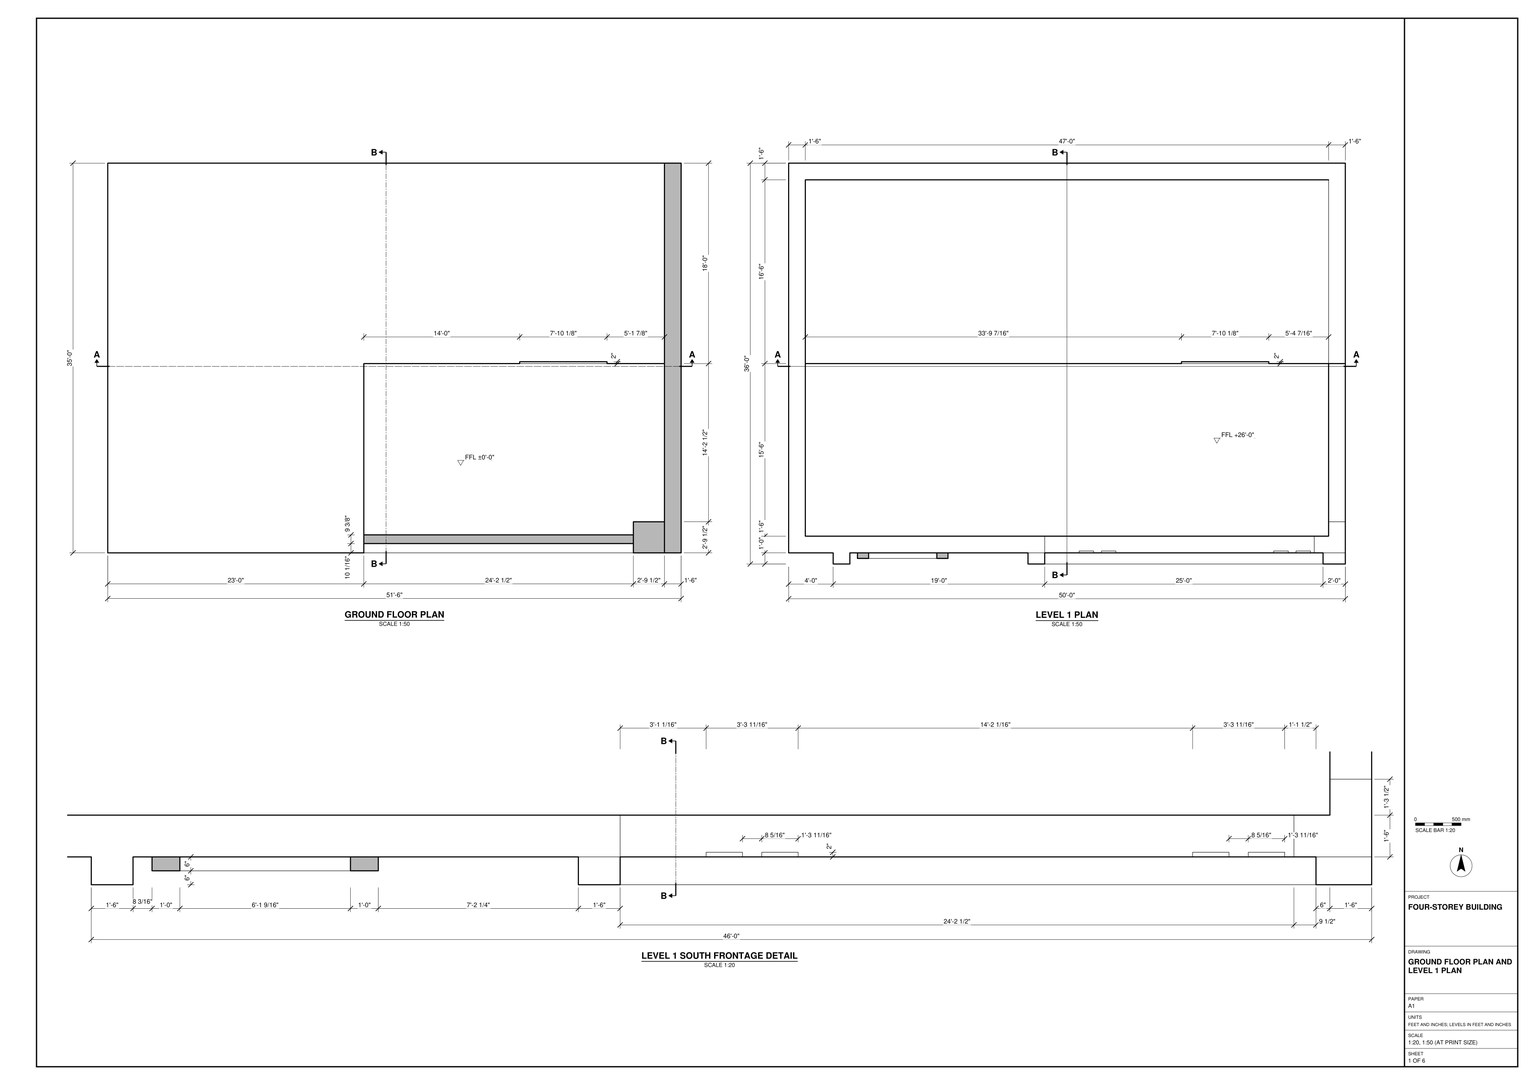
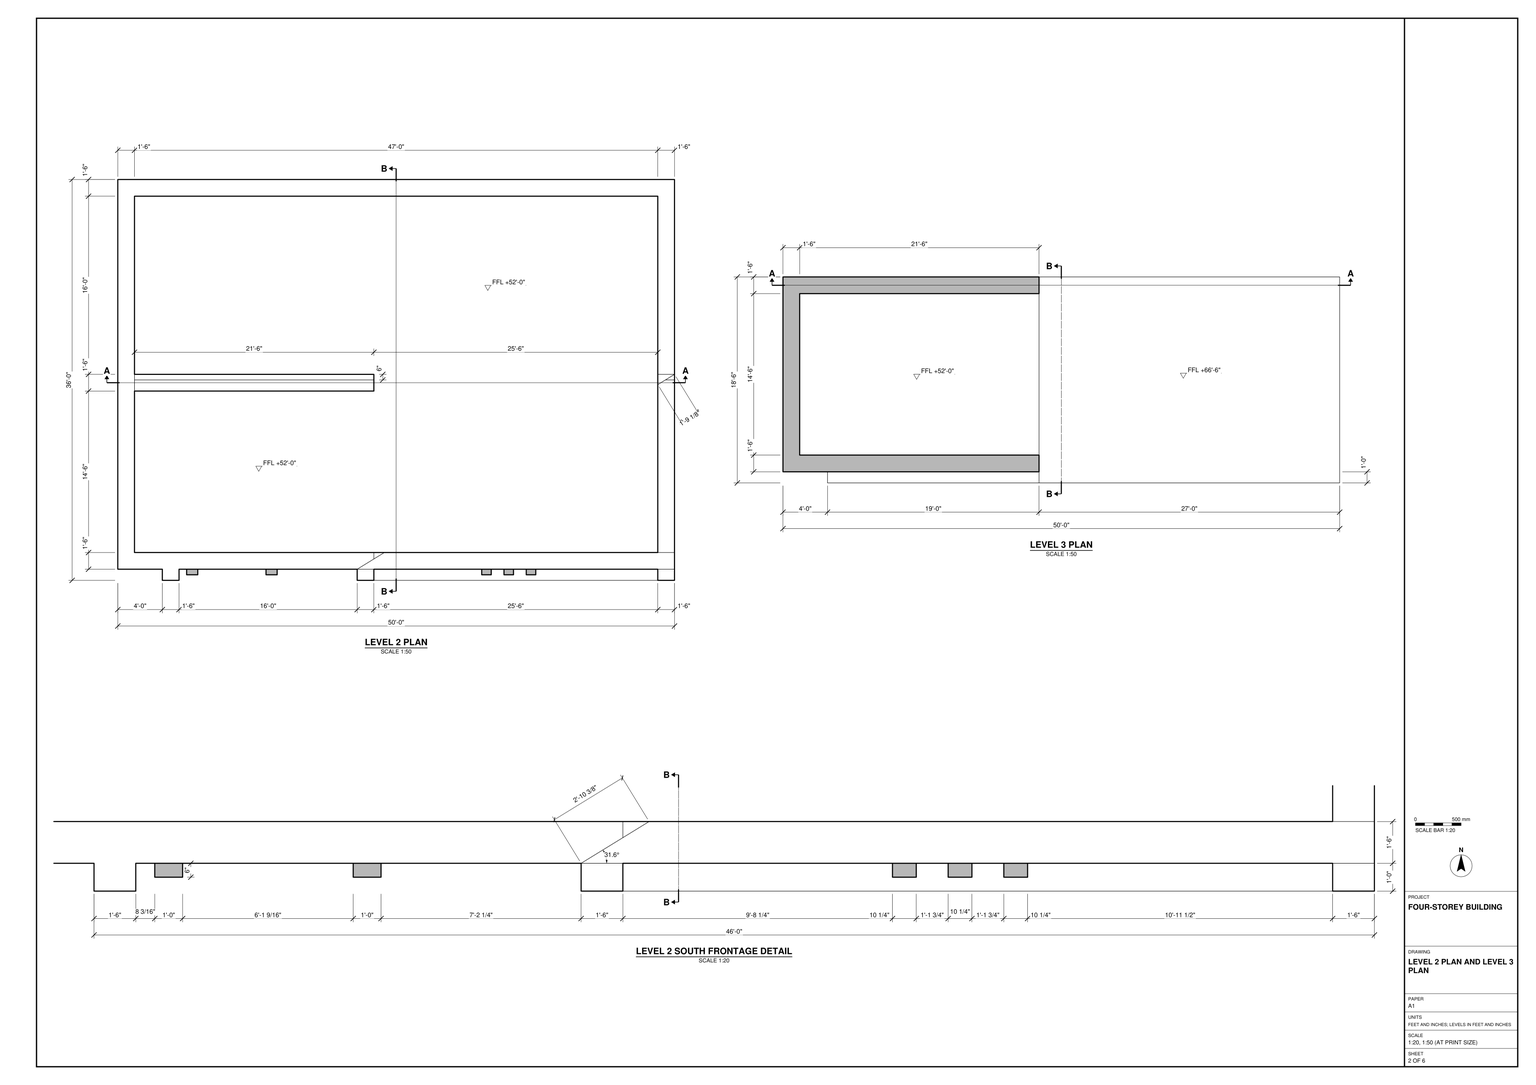
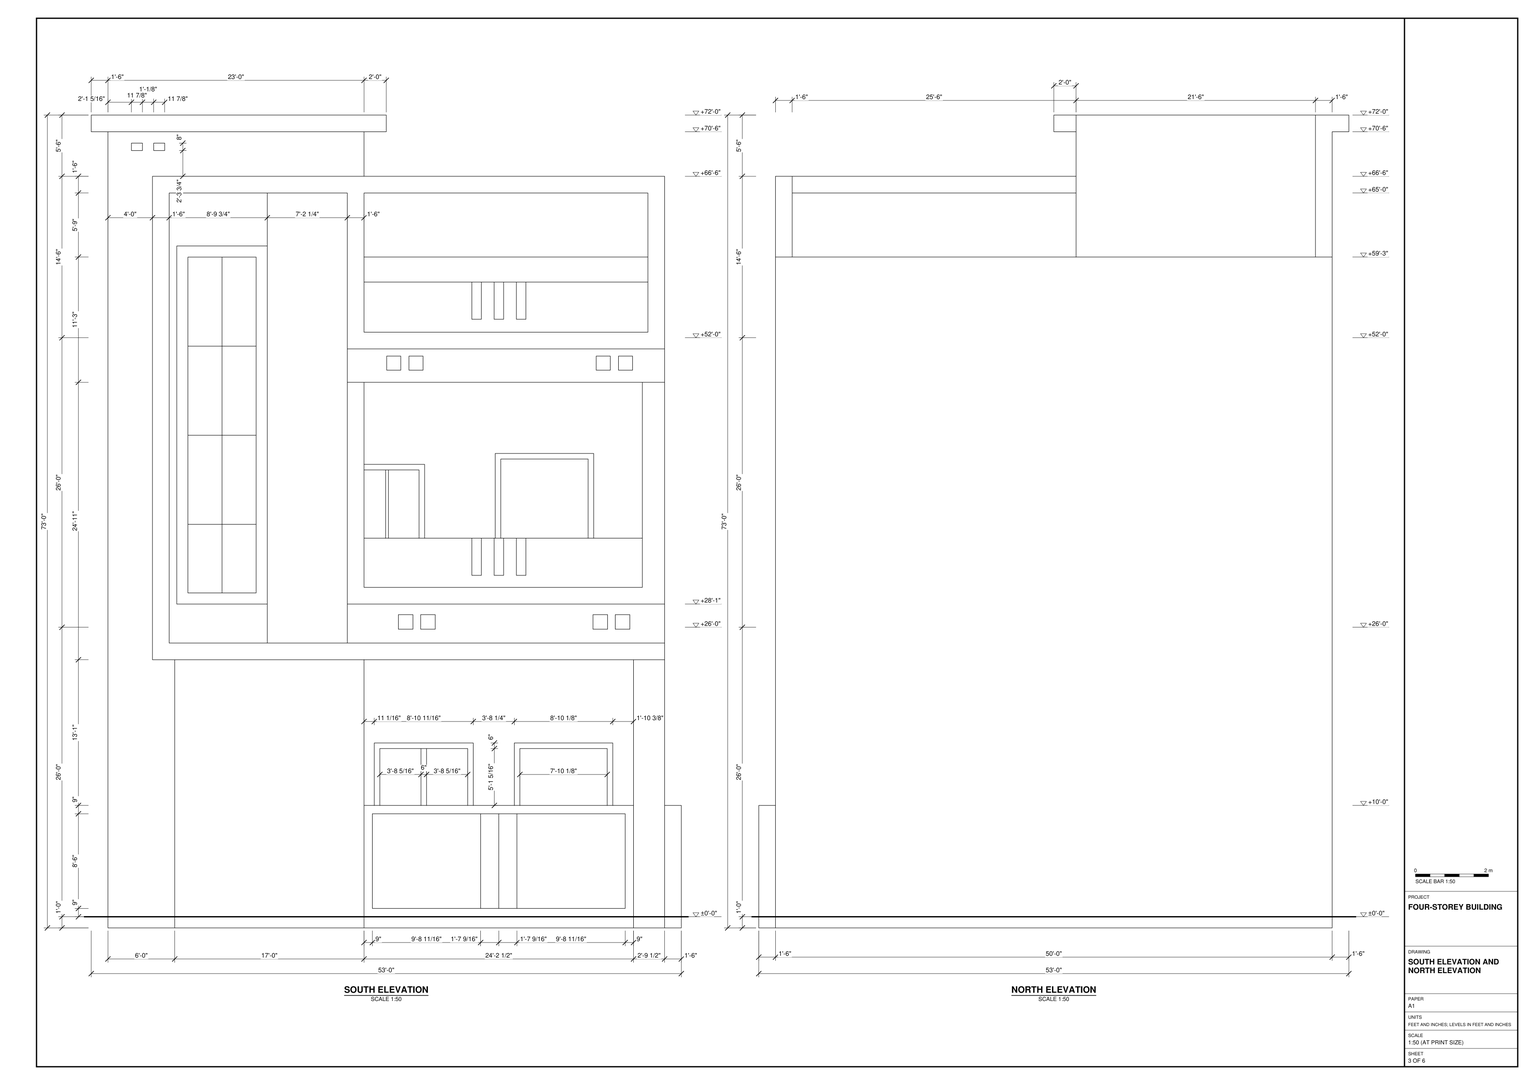
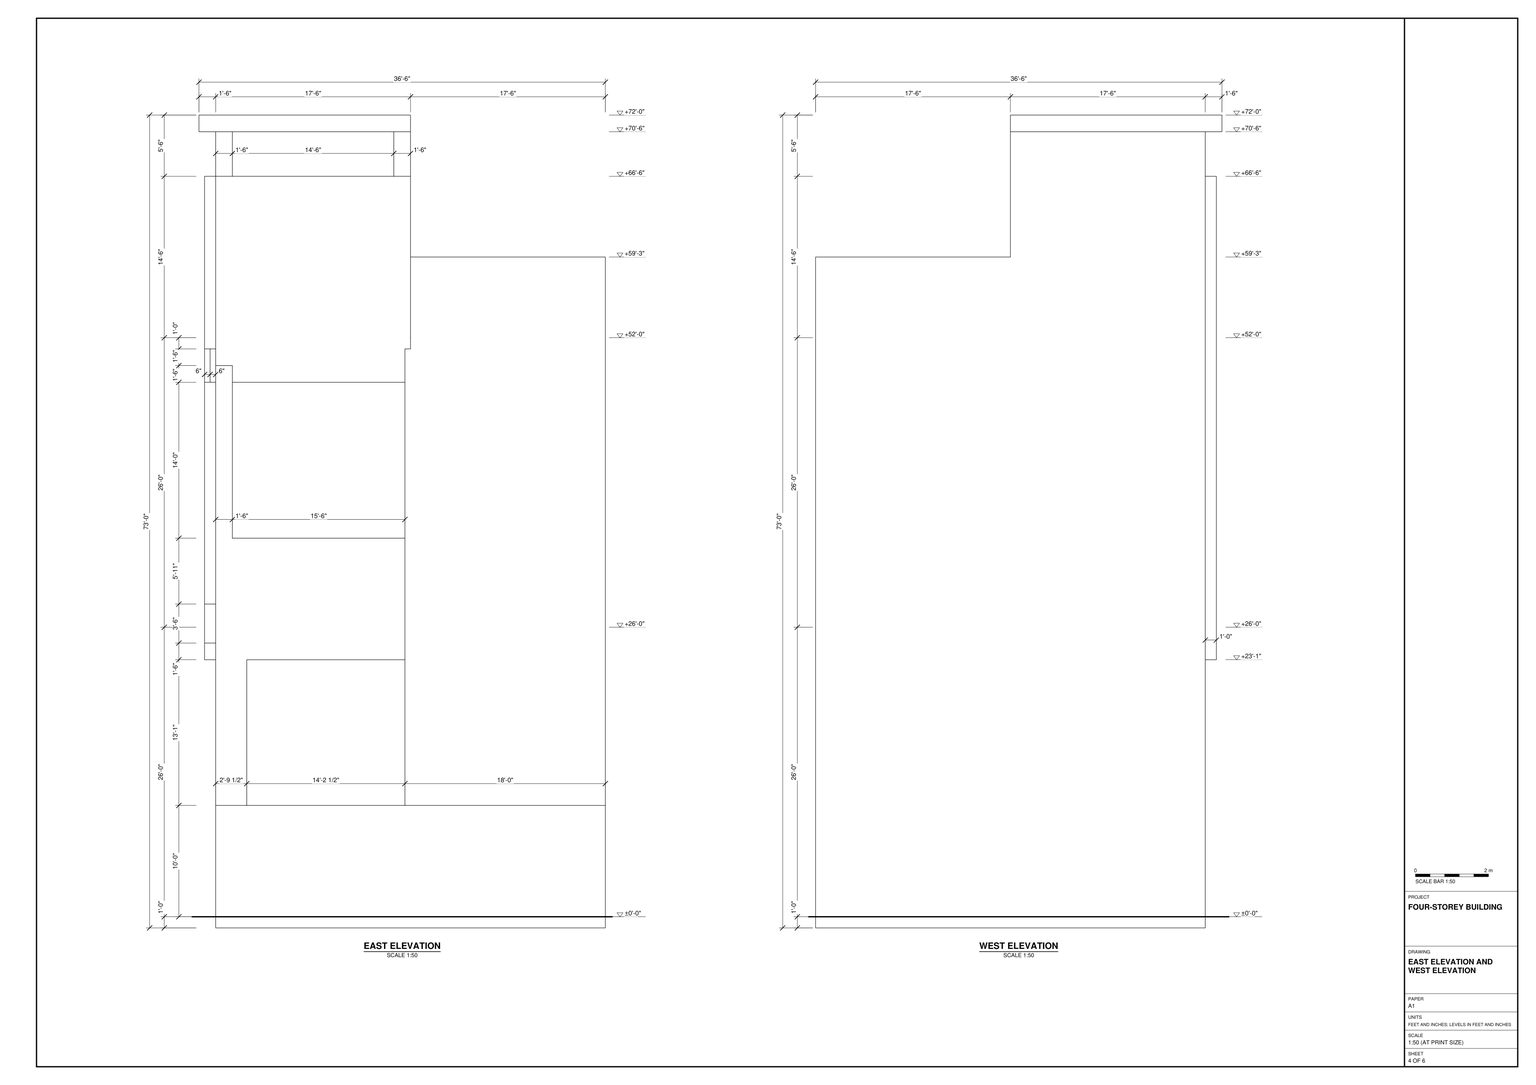
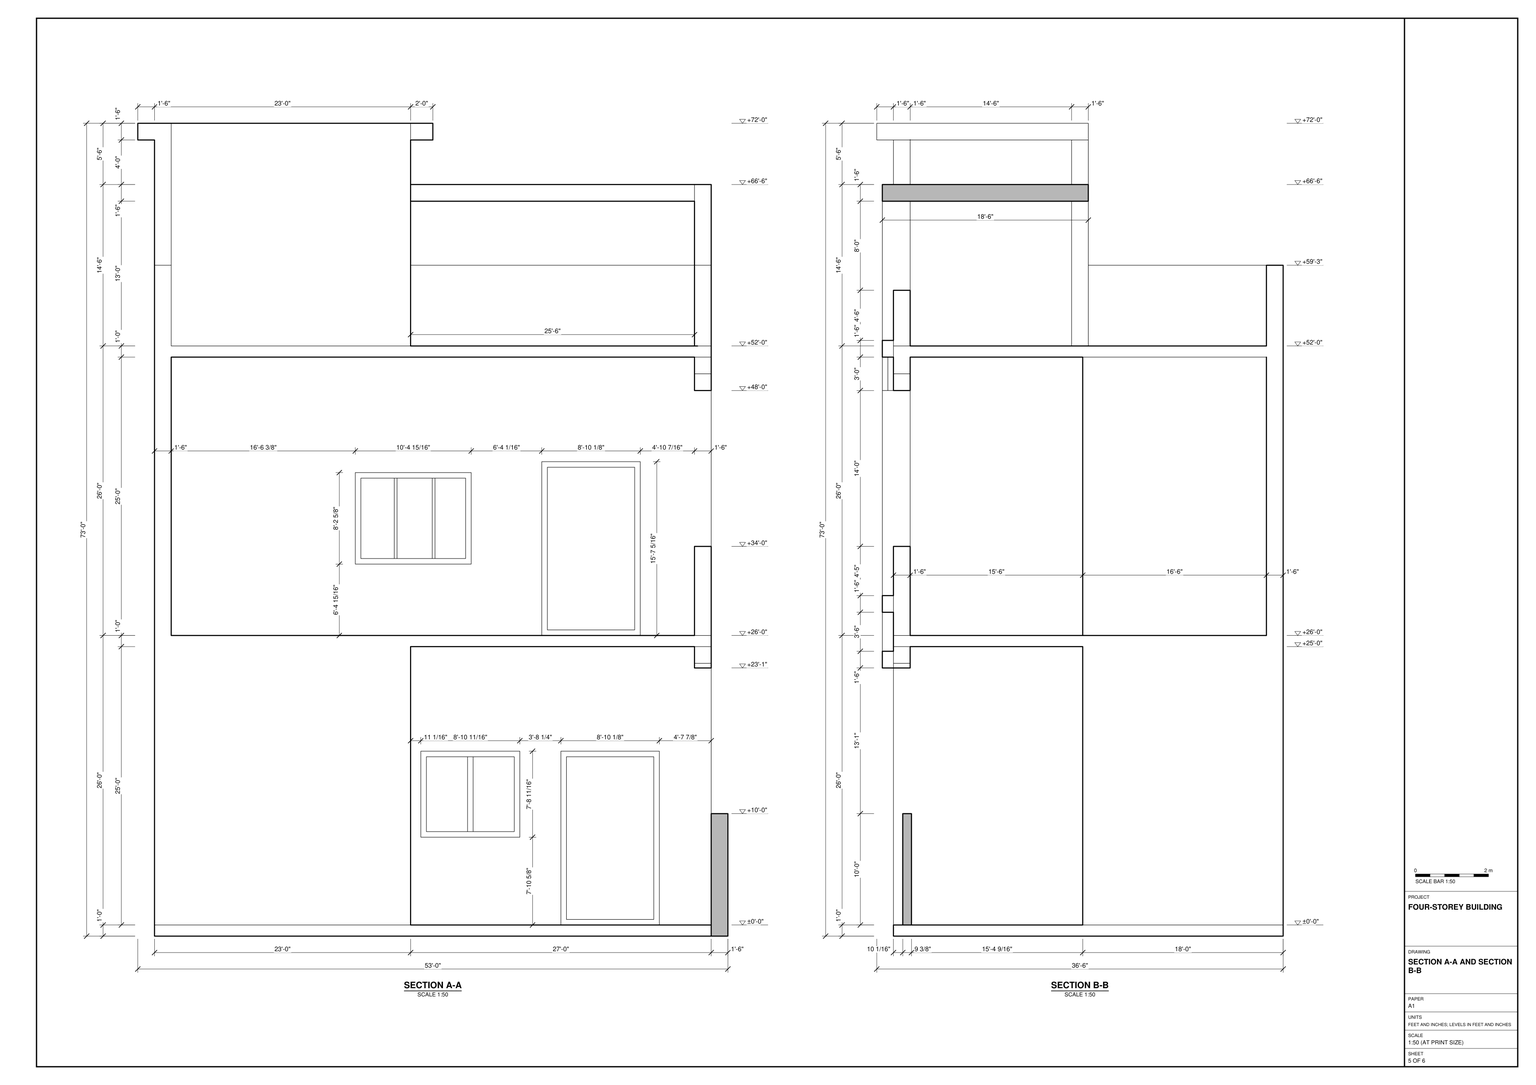
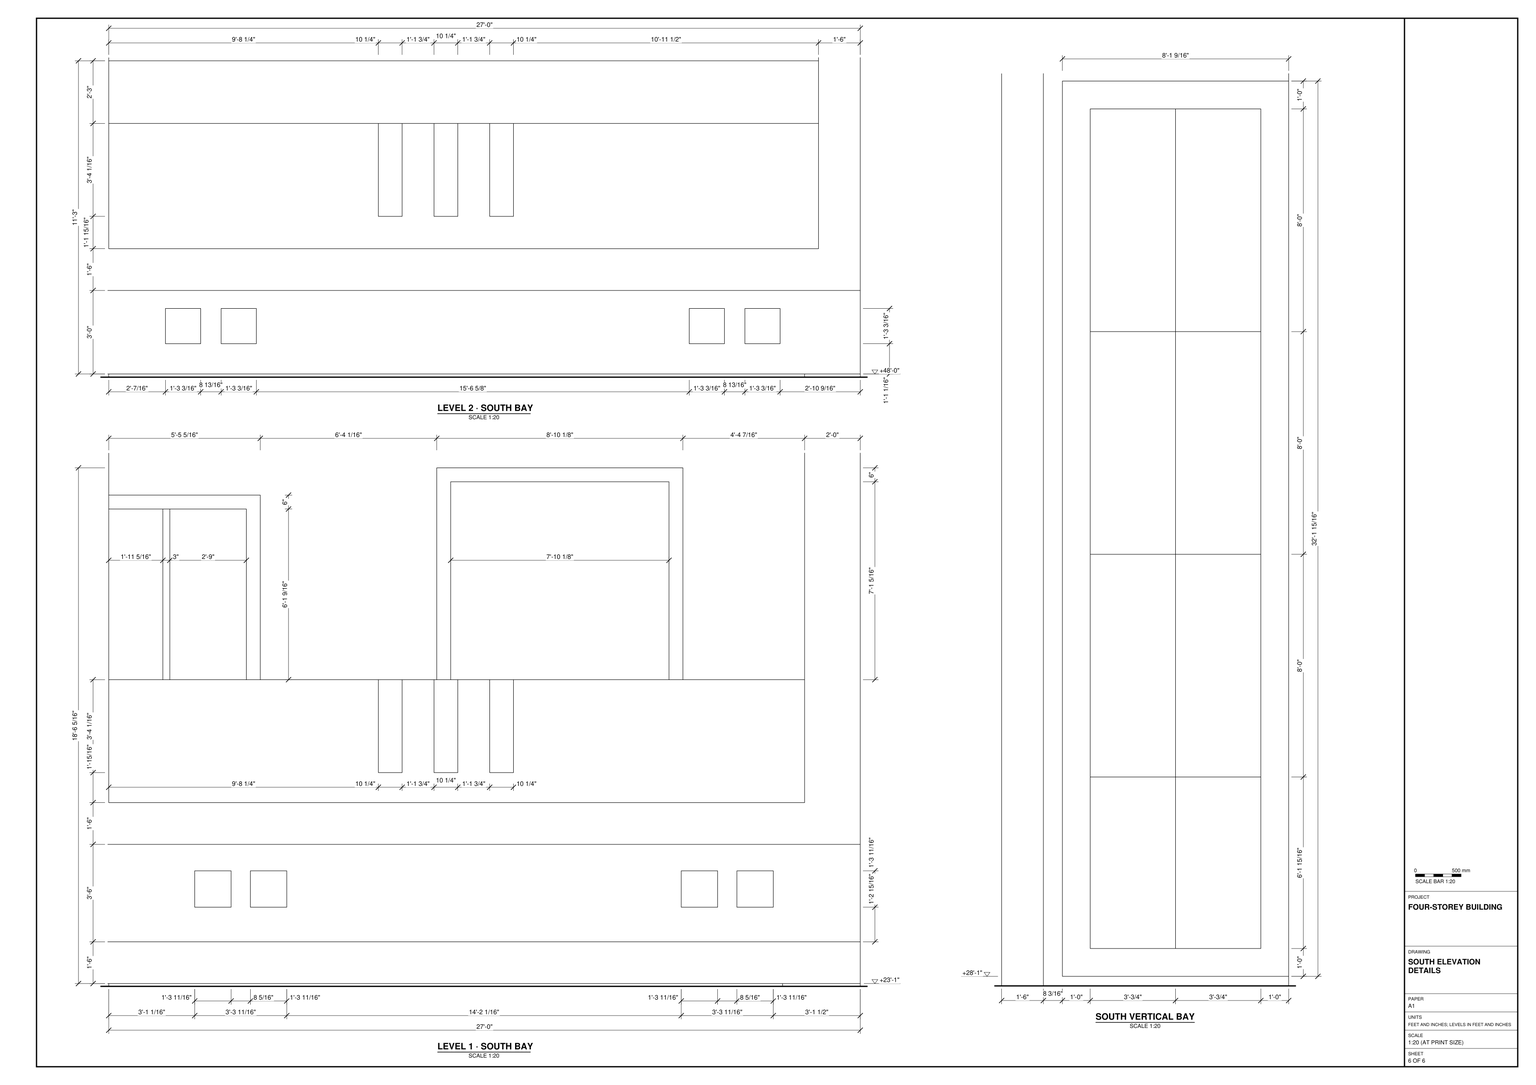
Build the four-storey building in SketchUp from task_files/diagram_01.pdf. Work in feet and inches. The overall model, including the base and roof projections, is 53'-0" wide, 36'-6" deep and 73'-0" high. Set the floor levels at ±0'-0", +26'-0", +52'-0" and +66'-6" relative to the ground floor.

Use the plans to lay out the base, floor slabs and walls, matching the wall thicknesses and offsets as drawn. Follow the frontage details to set the depth of the projecting frame and the recesses behind it. On the south elevation, model the low framed panels at ground level, the tall divided panel on the left and the stacked recessed bays on the right. Include the openings, low fronts and small square and vertical details in the positions shown. Keep the north wall plain below the roofline. Use the upper plan and elevations together to locate the raised western portion and its overhanging flat roof cap.

Keep walls, slabs and roof elements in separate groups or components, and do the same for each furniture or joinery piece shown. Use components for repeated parts. Decor and loose items may be any suitable library components. Save one SketchUp model as output_files/four_storey_building_with_a_framed_south_frontage.skp.

# SketchUp Ruby script. Lengths in inches.
U = 1.inch
M = Sketchup.active_model
def pt(a) = Geom::Point3d.new(a.map { |v| v * U })
def face(e, loops, mat)
  f = e.add_face(loops[0].map { |a| pt(a) })
  loops[1..].each { |l| e.add_face(l.map { |a| pt(a) }).erase! }
  f.material = f.back_material = mat if mat
  f
end
# faces: each face lists its corners as indices into pts; further lists are holes
def faces(e, pts, list, mat = nil) = list.each { |f| face(e, (f[0].is_a?(Array) ? f : [f]).map { |l| l.map { |i| pts[i] } }, mat) }
# xy, xz, yz: faces in a plane at the given z, y or x. An outline is a flat list of corners, or four numbers for a rectangle; further outlines are holes
def ring(l) = l.size == 4 ? [[l[0], l[1]], [l[2], l[1]], [l[2], l[3]], [l[0], l[3]]] : l.each_slice(2).to_a
def flat(e, list, mat, &to3) = list.each { |f| face(e, (f[0].is_a?(Array) ? f : [f]).map { |l| ring(l).map { |u, v| to3.(u, v) } }, mat) }
def xy(e, z, list, mat = nil) = flat(e, list, mat) { |x, y| [x, y, z] }
def xz(e, y, list, mat = nil) = flat(e, list, mat) { |x, z| [x, y, z] }
def yz(e, x, list, mat = nil) = flat(e, list, mat) { |y, z| [x, y, z] }
def lines(e, pts, list) = list.each { |a, b| e.add_line(pt(pts[a]), pt(pts[b])) }
# prism: a flat outline (further loops are holes) pulled along v
def prism(e, loops, v, mat = nil)
  f = face(e, loops, mat); d = Geom::Vector3d.new(v.map { |x| x * U })
  f.pushpull(f.normal.samedirection?(d) ? d.length : -d.length)
end
def box(e, o, s, mat = nil) = prism(e, [[o, [o[0] + s[0], o[1], o[2]], [o[0] + s[0], o[1] + s[1], o[2]], [o[0], o[1] + s[1], o[2]]]], [0, 0, s[2]], mat)
def at(x, y, z, deg = 0) = Geom::Transformation.translation(pt([x, y, z])) * Geom::Transformation.rotation(ORIGIN, Z_AXIS, deg.degrees)
def axes(o, x, y, z) = Geom::Transformation.new([*x, 0, *y, 0, *z, 0, *pt(o).to_a, 1])
def part(name) = M.definitions.add(name)
# library, detail: a bought-in or finely detailed component or shape, given as its bounding box
def library(name, o, s) = part(name).tap { |d| box(d.entities, o, s) }
def detail(e, o, s) = box(e.add_group.entities, o, s)
def put(e, d, t, mat = nil) = e.add_instance(d, t).tap { |i| i.material = mat if mat }
def group(e, t, mat = nil) = e.add_group.tap { |g| g.transformation = t; g.material = mat if mat }.entities
root = M.entities
M.materials.add("[0009_Linen]").color = [250, 240, 230]
M.materials.add("[0012_Bisque]").color = [211, 189, 162]
M.materials.add("[0012_Bisque]1").color = [221, 198, 170]
M.materials.add("[0012_Bisque]2").color = [201, 180, 154]
M.materials.add("[0033_NavajoWhite]").color = [198, 173, 134]
M.materials.add("[0111_SlateGray]").color = [71, 81, 91]
M.materials.add("[0111_SlateGray]1").color = [81, 92, 104]
M.materials.add("[0111_SlateGray]2").color = [65, 74, 84]
M.materials.add("[0137_Black]").color = [0, 0, 0]
M.materials.add("[Cladding Siding Tan]").color = [162, 138, 91]
M.materials.add("[Cladding Siding Tan]1").color = [162, 126, 95]
M.materials.add("[Grass Dark Green]").color = [106, 157, 55]
M.materials.add("[Stone Marble]").color = [143, 138, 136]
M.materials.add("[Translucent Resin Crush Gray]").color = [184, 184, 184]
M.materials["[Translucent Resin Crush Gray]"].alpha = 0.8
M.materials.add("[Translucent Resin Crush Gray]1").color = [184, 184, 184]
M.materials["[Translucent Resin Crush Gray]1"].alpha = 0.8
M.materials.add("[Wood Bamboo]").color = [177, 105, 43]
M.materials.add("[Wood Cherry Original]").color = [152, 86, 42]
M.materials.add("[Wood Veneer 01]").color = [120, 70, 37]
xy(root,0,[[18,18,618,438],[618,18,636,438]])
xy(root,12,[[294,28.04,584.5,37.41]])
xy(root,12,[[294,18,584.5,28.04],[294,37.41,584.5,37.41,584.5,51.5,618,51.5,618,222,294,222]],"[Stone Marble]")
xy(root,18,[[462,222,556.125,224]])
xy(root,132,[[618,18,636,438]],"[0009_Linen]")
xy(root,132,[[294,28.04,584.5,37.41]],"[0137_Black]")
xy(root,193.3125,[[462,222,556.125,224]])
xy(root,289,[[600,51.5,618,222]],"[0012_Bisque]1")
xy(root,289,[[66,6,66,18,294,18,294,36,584.5,36,584.5,18,618,18,618,6]],"[0111_SlateGray]")
xy(root,307,[[84,6,618,18]],"[0111_SlateGray]")
xy(root,312,[[294,36,294,222,600,222,600,51.5,584.5,51.5,584.5,36]])
xy(root,321.91,[[540.81,18,556.5,20]])
xy(root,321.91,[[331.06,18,346.75,20],[355.06,18,370.75,20],[564.81,18,580.5,20]],"[Wood Bamboo]")
xy(root,324,[[36,222,600,420]])
xy(root,324,[[36,36,600,222]],"[Grass Dark Green]")
xy(root,330,[[441.42,222,535.54,224]])
xy(root,337.6,[[540.81,18,556.5,20],[564.81,18,580.5,20]])
xy(root,337.6,[[331.06,18,346.75,20],[355.06,18,370.75,20]],"[Wood Bamboo]")
xy(root,349,[[92.19,12,189.74,18]])
xy(root,349,[[276,6,618,18]],"[0111_SlateGray]")
xy(root,361,[[104.19,12,177.74,18]],"[0111_SlateGray]2")
xy(root,367,[[294,6,594,18]],"[0111_SlateGray]")
xy(root,379.9375,[[410.24,12,420.49,18],[434.24,12,444.49,18],[458.24,12,468.49,18]],"[0111_SlateGray]1")
xy(root,420,[[294,18,594,36]],"[0012_Bisque]1")
xy(root,420,[[600,36,618,222]],"[0033_NavajoWhite]")
xy(root,420,[[410.24,12,420.49,18],[434.24,12,444.49,18],[458.24,12,468.49,18]],"[0111_SlateGray]1")
xy(root,505.3125,[[441.42,222,535.54,224]])
xy(root,588,[[[294,18,594,36],[361.58,20.98,363.125,21.21,364.5625,21.84,365.79,22.82,366.72,24.08,367.29,25.53,367.47,27.09,367.23,28.64,366.61,30.08,365.63,31.3,364.37,32.23,362.91,32.8,361.36,32.98,359.81,32.75,358.37,32.12,357.15,31.14,356.22,29.88,355.64,28.43,355.47,26.87,355.7,25.32,356.33,23.89,357.3,22.66,358.5625,21.73,360.02,21.16],[457.58,20.98,459.125,21.21,460.5625,21.84,461.79,22.82,462.72,24.08,463.29,25.53,463.47,27.09,463.23,28.64,462.61,30.08,461.63,31.3,460.37,32.23,458.91,32.8,457.36,32.98,455.81,32.75,454.37,32.12,453.15,31.14,452.22,29.88,451.64,28.43,451.47,26.87,451.7,25.32,452.33,23.89,453.3,22.66,454.5625,21.73,456.02,21.16],[553.58,20.98,555.125,21.21,556.5625,21.84,557.79,22.82,558.72,24.08,559.29,25.53,559.47,27.09,559.23,28.64,558.61,30.08,557.63,31.3,556.37,32.23,554.91,32.8,553.36,32.98,551.81,32.75,550.37,32.12,549.15,31.14,548.22,29.88,547.64,28.43,547.47,26.87,547.7,25.32,548.33,23.89,549.3,22.66,550.5625,21.73,552.02,21.16]],[361.58,20.98,360.02,21.16,358.5625,21.73,357.3,22.66,356.33,23.89,355.7,25.32,355.47,26.87,355.64,28.43,356.22,29.88,357.15,31.14,358.37,32.12,359.81,32.75,361.36,32.98,362.91,32.8,364.37,32.23,365.63,31.3,366.61,30.08,367.23,28.64,367.47,27.09,367.29,25.53,366.72,24.08,365.79,22.82,364.5625,21.84,363.125,21.21],[457.58,20.98,456.02,21.16,454.5625,21.73,453.3,22.66,452.33,23.89,451.7,25.32,451.47,26.87,451.64,28.43,452.22,29.88,453.15,31.14,454.37,32.12,455.81,32.75,457.36,32.98,458.91,32.8,460.37,32.23,461.63,31.3,462.61,30.08,463.23,28.64,463.47,27.09,463.29,25.53,462.72,24.08,461.79,22.82,460.5625,21.84,459.125,21.21],[553.58,20.98,552.02,21.16,550.5625,21.73,549.3,22.66,548.33,23.89,547.7,25.32,547.47,26.87,547.64,28.43,548.22,29.88,549.15,31.14,550.37,32.12,551.81,32.75,553.36,32.98,554.91,32.8,556.37,32.23,557.63,31.3,558.61,30.08,559.23,28.64,559.47,27.09,559.29,25.53,558.72,24.08,557.79,22.82,556.5625,21.84,555.125,21.21],[600,36,618,222]])
xy(root,588,[[276,6,294,18],[594,6,618,18]],"[0111_SlateGray]")
xy(root,601.05,[[318.45,18,333.64,20],[342.45,18,357.64,20],[544.26,18,559.45,20],[568.26,18,583.45,20]],"[Wood Bamboo]")
xy(root,616.24,[[318.45,18,333.64,20],[342.45,18,357.64,20],[544.26,18,559.45,20],[568.26,18,583.45,20]],"[Wood Bamboo]")
xy(root,624,[[36,36,600,222]])
xy(root,624,[[276,6,618,18]],"[0111_SlateGray]")
xy(root,636,[[294,29.05,305.3125,36,294,36],[600,216.95,600,228,618,228]])
xy(root,636,[[36,36,600,36,600,420,36,420,36,228,294,228,294,210,36,210]],"[0009_Linen]")
xy(root,642,[[294,6,600,18]],"[0111_SlateGray]")
xy(root,655.9375,[[410.24,12,420.49,18],[434.24,12,444.49,18],[458.24,12,468.49,18]],"[0111_SlateGray]1")
xy(root,696,[[294,18,600,36]],"[0012_Bisque]1")
xy(root,696,[[410.24,12,420.49,18],[434.24,12,444.49,18],[458.24,12,468.49,18]],"[0111_SlateGray]1")
xy(root,722.93,[[104.19,12,177.74,18]],"[0111_SlateGray]2")
xy(root,723,[[18,228,36,228,36,420,600,420,600,228,618,228,618,438,18,438]],"[0009_Linen]")
xy(root,734.93,[[92.19,12,189.74,18]],"[0111_SlateGray]2")
xy(root,792,[[343.01,70.9,339.97,71.67,337.24,73.21,335,75.39,333.4,78.09,332.55,81.1,332.51,84.23,333.28,87.27,334.8125,90,337,92.25,339.69,93.85,342.71,94.69,345.84,94.73,348.875,93.96,351.61,92.43,353.85,90.24,355.45,87.55,356.3,84.53,356.34,81.4,355.57,78.36,354.03,75.63,351.85,73.39,349.15,71.79,346.14,70.94],[439.01,70.9,435.97,71.67,433.24,73.21,431,75.39,429.4,78.09,428.55,81.1,428.51,84.23,429.28,87.27,430.8125,90,433,92.25,435.69,93.85,438.71,94.69,441.84,94.73,444.875,93.96,447.61,92.43,449.85,90.24,451.45,87.55,452.3,84.53,452.34,81.4,451.57,78.36,450.03,75.63,447.85,73.39,445.15,71.79,442.14,70.94],[535.01,70.9,531.97,71.67,529.24,73.21,527,75.39,525.4,78.09,524.55,81.1,524.51,84.23,525.28,87.27,526.8125,90,529,92.25,531.69,93.85,534.71,94.69,537.84,94.73,540.875,93.96,543.61,92.43,545.85,90.24,547.45,87.55,548.3,84.53,548.34,81.4,547.57,78.36,546.03,75.63,543.85,73.39,541.15,71.79,538.14,70.94]])
xy(root,792,[[84,6,276,18]],"[0111_SlateGray]1")
xy(root,792,[[[294,6,600,228],[343.01,70.9,346.14,70.94,349.15,71.79,351.85,73.39,354.03,75.63,355.57,78.36,356.34,81.4,356.3,84.53,355.45,87.55,353.85,90.24,351.61,92.43,348.875,93.96,345.84,94.73,342.71,94.69,339.69,93.85,337,92.25,334.8125,90,333.28,87.27,332.51,84.23,332.55,81.1,333.4,78.09,335,75.39,337.24,73.21,339.97,71.67],[439.01,70.9,442.14,70.94,445.15,71.79,447.85,73.39,450.03,75.63,451.57,78.36,452.34,81.4,452.3,84.53,451.45,87.55,449.85,90.24,447.61,92.43,444.875,93.96,441.84,94.73,438.71,94.69,435.69,93.85,433,92.25,430.8125,90,429.28,87.27,428.51,84.23,428.55,81.1,429.4,78.09,431,75.39,433.24,73.21,435.97,71.67],[535.01,70.9,538.14,70.94,541.15,71.79,543.85,73.39,546.03,75.63,547.57,78.36,548.34,81.4,548.3,84.53,547.45,87.55,545.85,90.24,543.61,92.43,540.875,93.96,537.84,94.73,534.71,94.69,531.69,93.85,529,92.25,526.8125,90,525.28,87.27,524.51,84.23,524.55,81.1,525.4,78.09,527,75.39,529.24,73.21,531.97,71.67]]],"[Wood Veneer 01]")
xy(root,810,[[294,6,618,228]],"[0009_Linen]")
xy(root,810,[[66,6,294,18]],"[0111_SlateGray]")
xy(root,837.75,[[43.32,18,55.2,20],[67.32,18,79.2,20]])
xy(root,845.75,[[43.32,18,55.2,20],[67.32,18,79.2,20]])
xy(root,858,[[306.19,33.7,304.64,33.91,303.19,34.51,301.95,35.46,301,36.7,300.4,38.15,300.19,39.7,300.4,41.25,301,42.7,301.95,43.94,303.19,44.9,304.64,45.5,306.19,45.7,307.75,45.5,309.19,44.9,310.4375,43.94,311.39,42.7,311.99,41.25,312.19,39.7,311.99,38.15,311.39,36.7,310.4375,35.46,309.19,34.51,307.75,33.91],[306.19,75.7,304.64,75.91,303.19,76.51,301.95,77.46,301,78.7,300.4,80.15,300.19,81.7,300.4,83.25,301,84.7,301.95,85.94,303.19,86.9,304.64,87.5,306.19,87.7,307.75,87.5,309.19,86.9,310.4375,85.94,311.39,84.7,311.99,83.25,312.19,81.7,311.99,80.15,311.39,78.7,310.4375,77.46,309.19,76.51,307.75,75.91],[306.19,117.7,304.64,117.91,303.19,118.51,301.95,119.46,301,120.7,300.4,122.15,300.19,123.7,300.4,125.25,301,126.7,301.95,127.94,303.19,128.9,304.64,129.5,306.19,129.7,307.75,129.5,309.19,128.9,310.4375,127.94,311.39,126.7,311.99,125.25,312.19,123.7,311.99,122.15,311.39,120.7,310.4375,119.46,309.19,118.51,307.75,117.91]])
xy(root,858,[[[0,0,0,228,18,228,18,18,294,18,294,36,36,36,36,210,294,210,294,228,318,228,318,0],[306.19,33.7,307.75,33.91,309.19,34.51,310.4375,35.46,311.39,36.7,311.99,38.15,312.19,39.7,311.99,41.25,311.39,42.7,310.4375,43.94,309.19,44.9,307.75,45.5,306.19,45.7,304.64,45.5,303.19,44.9,301.95,43.94,301,42.7,300.4,41.25,300.19,39.7,300.4,38.15,301,36.7,301.95,35.46,303.19,34.51,304.64,33.91],[306.19,75.7,307.75,75.91,309.19,76.51,310.4375,77.46,311.39,78.7,311.99,80.15,312.19,81.7,311.99,83.25,311.39,84.7,310.4375,85.94,309.19,86.9,307.75,87.5,306.19,87.7,304.64,87.5,303.19,86.9,301.95,85.94,301,84.7,300.4,83.25,300.19,81.7,300.4,80.15,301,78.7,301.95,77.46,303.19,76.51,304.64,75.91],[306.19,117.7,307.75,117.91,309.19,118.51,310.4375,119.46,311.39,120.7,311.99,122.15,312.19,123.7,311.99,125.25,311.39,126.7,310.4375,127.94,309.19,128.9,307.75,129.5,306.19,129.7,304.64,129.5,303.19,128.9,301.95,127.94,301,126.7,300.4,125.25,300.19,123.7,300.4,122.15,301,120.7,301.95,119.46,303.19,118.51,304.64,117.91]]],"[Wood Veneer 01]")
xy(root,876,[[0,0,318,228]],"[0009_Linen]")
xz(root,0,[[0,858,318,876]],"[0111_SlateGray]")
xz(root,6,[[[66,289,618,289,618,307,84,307,84,792,276,792,276,624,618,624,618,810,66,810],[294,642,600,792]],[276,349,618,349,618,588,594,588,594,367,294,367,294,588,276,588]],"[0111_SlateGray]")
xz(root,12,[[410.24,379.9375,420.49,420],[434.24,379.9375,444.49,420],[458.24,379.9375,468.49,420],[410.24,655.9375,420.49,696],[434.24,655.9375,444.49,696],
  [458.24,655.9375,468.49,696]],"[0111_SlateGray]1")
xz(root,12,[[[92.19,349,189.74,734.93],[104.19,361,177.74,722.93]]],"[0111_SlateGray]2")
xz(root,18,[[[92.19,349,189.74,734.93],[104.19,361,177.74,722.93]],[410.24,379.9375,420.49,420],[434.24,379.9375,444.49,420],[458.24,379.9375,468.49,420],[410.24,655.9375,420.49,696],
  [434.24,655.9375,444.49,696],[458.24,655.9375,468.49,696]])
xz(root,18,[[84,307,189.74,307,189.74,349,92.19,349,92.19,734.93,189.74,734.93,189.74,792,84,792],[[276,307,618,349],[540.81,321.91,556.5,337.6],[564.81,321.91,580.5,337.6],[355.06,321.91,370.75,337.6],[331.06,321.91,346.75,337.6]],[[276,588,618,624],[544.26,601.05,559.45,616.24],[568.26,601.05,583.45,616.24],[342.45,601.05,357.64,616.24],[318.45,601.05,333.64,616.24]]],"[0012_Bisque]")
xz(root,18,[[90,0,294,289],[584.5,0,618,289],[294,367,594,367,594,420,468.49,420,468.49,379.9375,458.24,379.9375,458.24,420,444.49,420,444.49,379.9375,434.24,379.9375,434.24,420,420.49,420,420.49,379.9375,410.24,379.9375,410.24,420,294,420],[294,642,600,642,600,696,468.49,696,468.49,655.9375,458.24,655.9375,458.24,696,444.49,696,444.49,655.9375,434.24,655.9375,434.24,696,420.49,696,420.49,655.9375,410.24,655.9375,410.24,696,294,696]],"[0012_Bisque]1")
xz(root,18,[[618,0,636,132]],"[0012_Bisque]2")
xz(root,18,[[[18,0,90,0,90,289,66,289,66,810,294,810,294,858,18,858],[43.32,837.75,55.2,845.75],[67.32,837.75,79.2,845.75]]],"[0033_NavajoWhite]")
xz(root,18,[[189.74,307,276,792]],"[Cladding Siding Tan]")
xz(root,18,[[294,0,584.5,12]],"[Stone Marble]")
xz(root,18,[[104.19,361,140.97,434.93],[140.97,361,177.74,434.93],[104.19,434.93,140.97,530.93],[140.97,434.93,177.74,530.93],[104.19,530.93,140.97,626.93],
  [140.97,530.93,177.74,626.93],[104.19,626.93,140.97,722.93],[140.97,626.93,177.74,722.93]],"[Translucent Resin Crush Gray]1")
xz(root,20,[[43.32,837.75,55.2,845.75],[67.32,837.75,79.2,845.75]])
xz(root,20,[[331.06,321.91,346.75,337.6],[355.06,321.91,370.75,337.6],[540.81,321.91,556.5,337.6],[564.81,321.91,580.5,337.6],[318.45,601.05,333.64,616.24],
  [342.45,601.05,357.64,616.24],[544.26,601.05,559.45,616.24],[568.26,601.05,583.45,616.24]],"[Wood Bamboo]")
xz(root,28.04,[[[294,12,584.5,132],[303,21,575.5,123]],[419.7,21,439.25,123],[439.25,21,458.8,123]],"[0137_Black]")
xz(root,28.04,[[303,21,419.7,123],[458.8,21,575.5,123]],"[Cladding Siding Tan]1")
xz(root,36,[[294,289,584.5,312],[594,420,594,606,600,606,600,588,618,588,618,420]])
xz(root,36,[[36,636,294,858],[294,636,600,696]],"[0012_Bisque]1")
xz(root,36,[[36,324,36,624,600,624,600,606,594,606,594,588,294,588,294,420,600,420,600,324]],"[0033_NavajoWhite]")
xz(root,37.41,[[294,12,584.5,132]])
xz(root,51.5,[[584.5,12,584.5,312,600,312,600,289,618,289,618,12]],"[0012_Bisque]1")
xz(root,210,[[36,636,294,858]],"[0012_Bisque]1")
xz(root,222,[[600,289,618,294],[600,294,618,312],[600,324,618,420],[600,588,618,606],[600,606,618,624]])
xz(root,222,[[[294,12,456,12,456,199.3125,562.125,199.3125,562.125,12,618,12,618,289,600,289,600,312,294,312],[305.06,106.625,411.75,199.3125]]],"[0012_Bisque]1")
xz(root,222,[[[36,324,435.42,324,435.42,511.3125,541.54,511.3125,541.54,324,600,324,600,420,618,420,618,588,600,588,600,624,36,624],[234.4,400.9375,359.33,499.5625]]],"[0033_NavajoWhite]")
xz(root,222,[[311.06,112.625,355.4,193.3125],[361.4,112.625,405.75,193.3125],[240.4,406.9375,276.4,493.5625],[279.4,406.9375,317.33,493.5625],[320.33,406.9375,353.33,493.5625]],"[Translucent Resin Crush Gray]")
xz(root,222,[[[305.06,106.625,411.75,199.3125],[311.06,112.625,405.75,193.3125]],[355.4,112.625,361.4,193.3125],[[234.4,400.9375,359.33,499.5625],[240.4,406.9375,353.33,493.5625]],[276.4,406.9375,279.4,493.5625],[317.33,406.9375,320.33,493.5625]],"[Wood Cherry Original]")
xz(root,222,[[[456,12,562.125,199.3125],[462,18,556.125,193.3125]],[[435.42,324,541.54,511.3125],[441.42,330,535.54,505.3125]]],"[Wood Veneer 01]")
xz(root,224,[[462,18,556.125,193.3125],[441.42,330,535.54,505.3125]],"[Wood Veneer 01]")
xz(root,228,[[600,723,618,810]])
xz(root,228,[[36,636,294,876],[294,792,600,810],[294,858,318,876]],"[0009_Linen]")
xz(root,228,[[18,723,18,858,0,858,0,876,36,876,36,723]],"[0111_SlateGray]")
xz(root,420,[[36,324,600,624]])
xz(root,420,[[36,636,600,723]],"[0012_Bisque]2")
xz(root,438,[[18,0,618,12],[618,0,636,12],[618,12,636,132]])
xz(root,438,[[18,12,618,723]],"[0009_Linen]")
yz(root,0,[[0,858,228,876]],"[0111_SlateGray]")
yz(root,18,[[18,0,438,12]])
yz(root,18,[[18,12,18,858,228,858,228,723,438,723,438,12]],"[0009_Linen]")
yz(root,36,[[222,324,420,624],[228,636,420,723]])
yz(root,36,[[36,636,210,858]],"[0012_Bisque]1")
yz(root,36,[[36,324,222,624]],"[0033_NavajoWhite]")
yz(root,43.32,[[18,837.75,20,845.75]])
yz(root,55.2,[[18,837.75,20,845.75]])
yz(root,66,[[6,289,18,810]],"[0111_SlateGray]")
yz(root,67.32,[[18,837.75,20,845.75]])
yz(root,79.2,[[18,837.75,20,845.75]])
yz(root,84,[[6,307,18,792]],"[0111_SlateGray]1")
yz(root,92.19,[[12,349,18,734.93]],"[0111_SlateGray]2")
yz(root,104.19,[[12,361,18,722.93]],"[0111_SlateGray]2")
yz(root,177.74,[[12,361,18,722.93]],"[0111_SlateGray]2")
yz(root,189.74,[[12,349,18,734.93]],"[0111_SlateGray]2")
yz(root,276,[[6,349,18,588],[6,624,18,792]],"[0111_SlateGray]")
yz(root,294,[[28.04,12,37.41,132],[18,792,36,810],[36,792,210,810],[210,792,228,810]])
yz(root,294,[[18,12,28.04,12,28.04,132,37.41,132,37.41,12,222,12,222,312,36,312,36,289,18,289],[18,810,36,858]],"[0012_Bisque]1")
yz(root,294,[[210,636,228,792],[210,810,228,858]],"[0012_Bisque]2")
yz(root,294,[[6,367,18,367,18,420,36,420,36,588,6,588],[6,642,18,642,18,696,36,696,36,792,6,792]],"[0111_SlateGray]")
yz(root,318,[[0,858,228,876]],"[0111_SlateGray]")
yz(root,318.45,[[18,601.05,20,616.24]],"[Wood Bamboo]")
yz(root,331.06,[[18,321.91,20,337.6]],"[Wood Bamboo]")
yz(root,333.64,[[18,601.05,20,616.24]],"[Wood Bamboo]")
yz(root,342.45,[[18,601.05,20,616.24]],"[Wood Bamboo]")
yz(root,346.75,[[18,321.91,20,337.6]],"[Wood Bamboo]")
yz(root,355.06,[[18,321.91,20,337.6]],"[Wood Bamboo]")
yz(root,357.64,[[18,601.05,20,616.24]],"[Wood Bamboo]")
yz(root,370.75,[[18,321.91,20,337.6]],"[Wood Bamboo]")
yz(root,410.24,[[12,379.9375,18,420],[12,655.9375,18,696]],"[0111_SlateGray]1")
yz(root,420.49,[[12,379.9375,18,420],[12,655.9375,18,696]],"[0111_SlateGray]1")
yz(root,434.24,[[12,379.9375,18,420],[12,655.9375,18,696]],"[0111_SlateGray]1")
yz(root,441.42,[[222,330,224,505.3125]])
yz(root,444.49,[[12,379.9375,18,420],[12,655.9375,18,696]],"[0111_SlateGray]1")
yz(root,458.24,[[12,379.9375,18,420],[12,655.9375,18,696]],"[0111_SlateGray]1")
yz(root,462,[[222,18,224,193.3125]])
yz(root,468.49,[[12,379.9375,18,420],[12,655.9375,18,696]],"[0111_SlateGray]1")
yz(root,535.54,[[222,330,224,505.3125]])
yz(root,540.81,[[18,321.91,20,337.6]])
yz(root,544.26,[[18,601.05,20,616.24]],"[Wood Bamboo]")
yz(root,556.125,[[222,18,224,193.3125]])
yz(root,556.5,[[18,321.91,20,337.6]])
yz(root,559.45,[[18,601.05,20,616.24]],"[Wood Bamboo]")
yz(root,564.81,[[18,321.91,20,337.6]])
yz(root,568.26,[[18,601.05,20,616.24]],"[Wood Bamboo]")
yz(root,580.5,[[18,321.91,20,337.6]])
yz(root,583.45,[[18,601.05,20,616.24]],"[Wood Bamboo]")
yz(root,584.5,[[28.04,12,37.41,132]])
yz(root,584.5,[[18,12,18,289,36,289,36,312,51.5,312,51.5,12,37.41,12,37.41,132,28.04,132,28.04,12]],"[0012_Bisque]1")
yz(root,594,[[18,420,36,588]],"[0033_NavajoWhite]")
yz(root,594,[[6,367,18,588]],"[0111_SlateGray]")
yz(root,600,[[36,588,222,624]])
yz(root,600,[[51.5,289,222,312]],"[0012_Bisque]1")
yz(root,600,[[36,324,222,420],[36,636,36,792,228,792,228,723,420,723,420,636]],"[0033_NavajoWhite]")
yz(root,600,[[6,642,6,792,36,792,36,696,18,696,18,642]],"[0111_SlateGray]")
yz(root,618,[[18,0,438,12],[18,12,51.5,132],[222,12,438,132]])
yz(root,618,[[51.5,12,222,132],[222,132,438,132,438,723,228,723,228,624,222,624],[36,588,222,588,222,624,228,624,228,810,18,810,18,606,36,606],[6,624,18,810]],"[0009_Linen]")
yz(root,618,[[18,132,51.5,132,51.5,289,222,289,222,420,36,420,36,606,18,606]],"[0033_NavajoWhite]")
yz(root,618,[[6,289,18,307],[6,349,18,588]],"[0111_SlateGray]")
yz(root,636,[[18,0,438,12],[18,12,438,132]],"[0009_Linen]")
p = [[294,36,324],[294,18,324],[36,36,858],[36,36,876],[36,210,858],[36,210,876],
  [600,36,636],[618,36,636],[600,36,792],[600,36,810],[600,420,624],[600,222,624],
  [294,36,312],[294,18,312],[600,51.5,312],[618,51.5,312],[584.5,18,312],[584.5,36,312],
  [294,36,294],[294,18,294],[584.5,18,294],[584.5,36,294],[600,51.5,294],[618,51.5,294],
  [594,18,606],[594,36,606],[294,36,606],[294,18,606],[294,29.05,636],[276,18,636]]
lines(root,p,[[0,1],[2,3],[4,5],[6,7],[8,9],[10,11],[12,13],[14,15],[16,17],[18,19],[20,21],[22,23],
  [24,25],[26,27],[28,29]])
